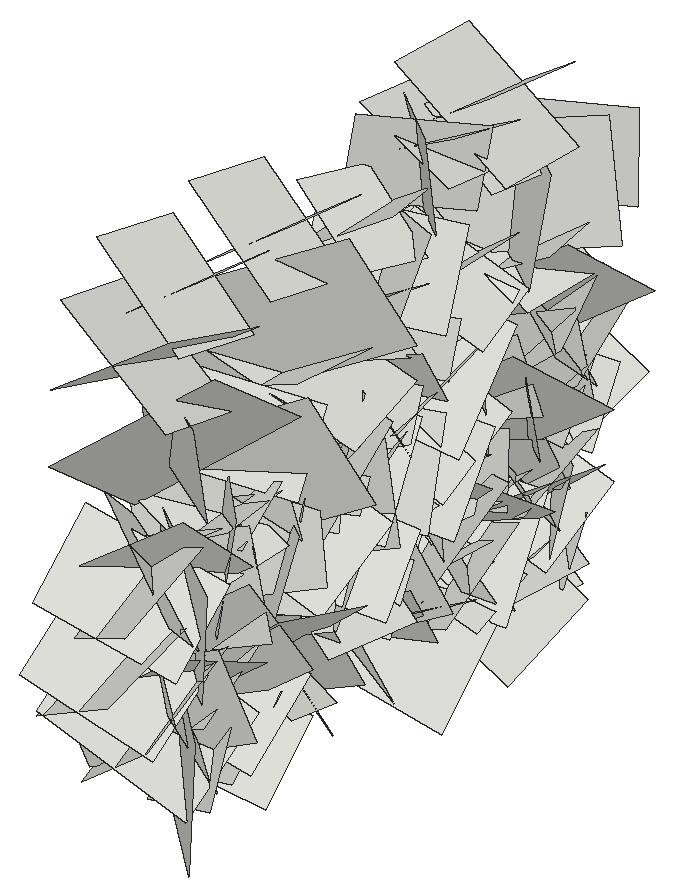
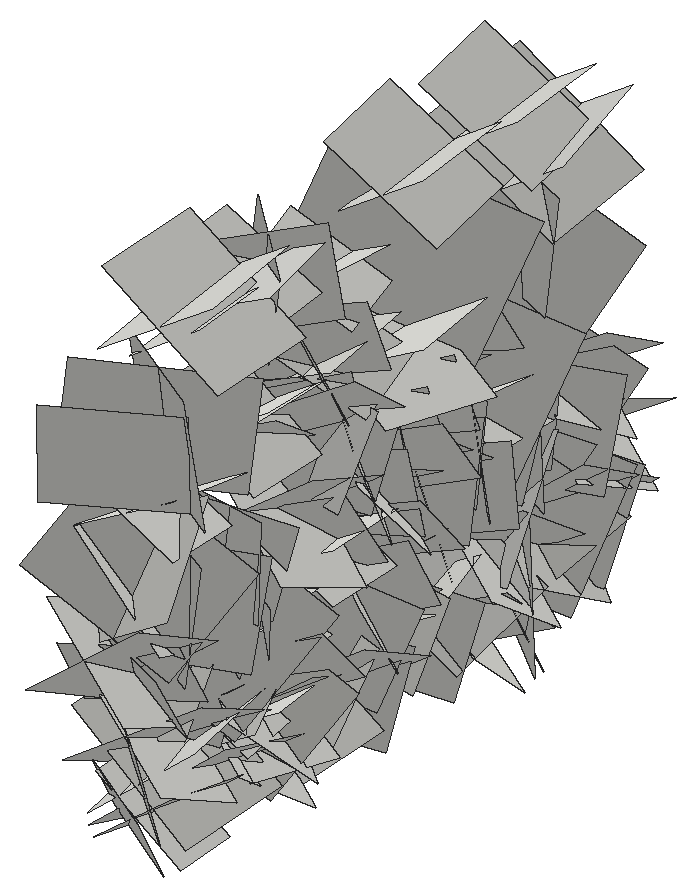
# SketchUp Ruby script. Lengths in inches.
U = 1.inch
M = Sketchup.active_model
def pt(a) = Geom::Point3d.new(a.map { |v| v * U })
def face(e, loops, mat)
  f = e.add_face(loops[0].map { |a| pt(a) })
  loops[1..].each { |l| e.add_face(l.map { |a| pt(a) }).erase! }
  f.material = f.back_material = mat if mat
  f
end
# faces: each face lists its corners as indices into pts; further lists are holes
def faces(e, pts, list, mat = nil) = list.each { |f| face(e, (f[0].is_a?(Array) ? f : [f]).map { |l| l.map { |i| pts[i] } }, mat) }
# xy, xz, yz: faces in a plane at the given z, y or x. An outline is a flat list of corners, or four numbers for a rectangle; further outlines are holes
def ring(l) = l.size == 4 ? [[l[0], l[1]], [l[2], l[1]], [l[2], l[3]], [l[0], l[3]]] : l.each_slice(2).to_a
def flat(e, list, mat, &to3) = list.each { |f| face(e, (f[0].is_a?(Array) ? f : [f]).map { |l| ring(l).map { |u, v| to3.(u, v) } }, mat) }
def xy(e, z, list, mat = nil) = flat(e, list, mat) { |x, y| [x, y, z] }
def xz(e, y, list, mat = nil) = flat(e, list, mat) { |x, z| [x, y, z] }
def yz(e, x, list, mat = nil) = flat(e, list, mat) { |y, z| [x, y, z] }
def lines(e, pts, list) = list.each { |a, b| e.add_line(pt(pts[a]), pt(pts[b])) }
# prism: a flat outline (further loops are holes) pulled along v
def prism(e, loops, v, mat = nil)
  f = face(e, loops, mat); d = Geom::Vector3d.new(v.map { |x| x * U })
  f.pushpull(f.normal.samedirection?(d) ? d.length : -d.length)
end
def box(e, o, s, mat = nil) = prism(e, [[o, [o[0] + s[0], o[1], o[2]], [o[0] + s[0], o[1] + s[1], o[2]], [o[0], o[1] + s[1], o[2]]]], [0, 0, s[2]], mat)
def at(x, y, z, deg = 0) = Geom::Transformation.translation(pt([x, y, z])) * Geom::Transformation.rotation(ORIGIN, Z_AXIS, deg.degrees)
def axes(o, x, y, z) = Geom::Transformation.new([*x, 0, *y, 0, *z, 0, *pt(o).to_a, 1])
def part(name) = M.definitions.add(name)
# library, detail: a bought-in or finely detailed component or shape, given as its bounding box
def library(name, o, s) = part(name).tap { |d| box(d.entities, o, s) }
def detail(e, o, s) = box(e.add_group.entities, o, s)
def put(e, d, t, mat = nil) = e.add_instance(d, t).tap { |i| i.material = mat if mat }
def group(e, t, mat = nil) = e.add_group.tap { |g| g.transformation = t; g.material = mat if mat }.entities
root = M.entities
c1 = part("Component\#6")
p = [[0.01,0,0],[0,3.24,4.54],[4.32,3.24,4.54],[4.33,0,0]]
faces(c1.entities,p,[[0,1,2,3]])
put(root,c1,axes([400.91,128.06,26.23],[-0.10092,-0.80547,-0.37503],[-0.00485,-0.37672,0.81027],[0.94179,-0.08825,-0.03602]))
put(root,c1,axes([404.88,128.06,26.23],[0.10092,-0.80547,-0.37503],[0.00485,-0.37672,0.81027],[-0.94179,-0.08825,-0.03602]))
put(root,c1,axes([400.91,129.13,29.07],[-0.11411,-0.79222,-0.47459],[-0.01099,-0.47673,0.79815],[0.97884,-0.0977,-0.04636]))
put(root,c1,axes([404.88,129.13,29.07],[0.11411,-0.79222,-0.47459],[0.01099,-0.47673,0.79815],[-0.97884,-0.0977,-0.04636]))
put(root,c1,axes([400.91,126.77,21.87],[-0.10992,-0.34124,0.92241],[0.05569,0.92428,0.34784],[1.04103,-0.08548,0.07879]))
put(root,c1,axes([400.91,129.34,35.47],[-0.09463,-0.94647,0.23979],[-0.00571,0.24126,0.95028],[1.03494,-0.08521,0.02717]))
put(root,c1,axes([404.88,129.34,35.47],[0.09463,-0.94647,0.23979],[0.00571,0.24126,0.95028],[-1.03494,-0.08521,0.02717]))
put(root,c1,axes([400.91,130.61,23.63],[-0.04049,-0.92661,-0.53015],[-0.18829,-0.51758,0.91743],[1.11583,-0.12096,0.13557]))
put(root,c1,axes([404.88,130.61,23.63],[0.04049,-0.92661,-0.53015],[0.18829,-0.51758,0.91743],[-1.11583,-0.12096,0.13557]))
put(root,c1,axes([400.91,128.14,26.625],[-0.13018,-0.67547,0.62862],[-0.07474,0.63918,0.67304],[0.97523,-0.04118,0.13549]))
put(root,c1,axes([404.88,128.14,26.625],[0.13018,-0.67547,0.62862],[0.07474,0.63918,0.67304],[-0.97523,-0.04118,0.13549]))
put(root,c1,axes([404.88,126.29,27.49],[0.18614,0.86586,-0.34095],[0.04817,-0.35453,-0.87695],[-0.98523,0.14625,-0.10729]))
put(root,c1,axes([400.91,129.02,36.97],[-0.03047,0.19902,-0.90037],[0.05941,-0.89877,-0.20045],[0.97562,0.06094,-0.01591]))
put(root,c1,axes([400.91,130.54,26.21],[-0.16316,0.13144,-1.2549],[-0.21583,-1.25022,-0.10597],[1.31994,-0.18819,-0.17245]))
put(root,c1,axes([400.91,129.15,30.625],[-0.089,-0.93417,0.70597],[-0.20388,0.70917,0.91554],[1.22433,0.05019,0.20378]))
put(root,c1,axes([400.91,130.09,30.86],[-0.13772,0.10296,-1.023],[-0.01142,-1.03121,-0.10242],[1.08979,0.0022,-0.13035]))
put(root,c1,axes([404.88,130.09,30.86],[0.13772,0.10296,-1.023],[0.01142,-1.03121,-0.10242],[-1.08979,0.0022,-0.13035]))
put(root,c1,axes([400.91,130.39,37.85],[0.05885,-0.83818,0.13983],[-0.03078,0.13818,0.83979],[0.90022,0.05952,0.01957]))
put(root,c1,axes([404.88,130.39,37.85],[-0.05885,-0.83818,0.13983],[0.03078,0.13818,0.83979],[-0.90022,0.05952,0.01957]))
put(root,c1,axes([400.91,128.44,21.53],[-0.07533,-0.68545,1.00594],[-0.30491,0.98857,0.65329],[1.25377,0.19923,0.21932]))
put(root,c1,axes([404.88,128.44,21.53],[0.07533,-0.68545,1.00594],[0.30491,0.98857,0.65329],[-1.25377,0.19923,0.21932]))
put(root,c1,axes([400.91,131.26,22.93],[0.10206,-0.4663,-0.72841],[0.02316,-0.73136,0.47108],[0.91647,0.07041,0.06921]))
put(root,c1,axes([404.88,127.73,24.28],[0.02979,0.75993,0.53946],[0.00151,0.53967,-0.7603],[-0.98786,0.02374,0.0151]))
put(root,c1,axes([400.91,127.73,24.28],[-0.02979,0.75993,0.53946],[-0.00151,0.53967,-0.7603],[0.98786,0.02374,0.0151]))
put(root,c1,axes([400.91,129.03,31.05],[0.04043,0.74356,0.04678],[0.07255,0.04314,-0.74161],[0.78639,-0.04221,0.06601]))
put(root,c1,axes([404.88,129.03,31.05],[-0.04043,0.74356,0.04678],[-0.07255,0.04314,-0.74161],[-0.78639,-0.04221,0.06601]))
put(root,c1,axes([400.91,133.52,31.89],[-0.15087,-0.04242,-1.05475],[-0.23169,-1.04005,0.07132],[1.09469,-0.22597,-0.13027]))
put(root,c1,axes([404.88,133.52,31.89],[0.15087,-0.04242,-1.05475],[0.23169,-1.04005,0.07132],[-1.09469,-0.22597,-0.13027]))
put(root,c1,axes([400.91,129.22,21.54],[-0.01805,0.58513,0.55019],[0.06792,0.54955,-0.58247],[0.84865,-0.03153,0.05832]))
put(root,c1,axes([404.88,129.22,21.54],[0.01805,0.58513,0.55019],[-0.06792,0.54955,-0.58247],[-0.84865,-0.03153,0.05832]))
put(root,c1,axes([404.88,129.75,30.06],[-0.01937,0.49926,0.36665],[-0.0577,0.36409,-0.4985],[-0.65405,-0.04691,0.03312]))
put(root,c1,axes([400.91,130.92,26.67],[-0.06799,-0.20959,0.7931],[0.02884,0.79454,0.21217],[0.86907,-0.04277,0.05501]))
put(root,c1,axes([404.88,130.92,26.67],[0.06799,-0.20959,0.7931],[-0.02884,0.79454,0.21217],[-0.86907,-0.04277,0.05501]))
put(root,c1,axes([400.91,131.21,27.63],[-0.2234,-0.54463,1.08834],[-0.02633,1.10624,0.54877],[1.28976,-0.07175,0.19972]))
put(root,c1,axes([404.88,134.18,33.55],[0.07538,-0.44425,-0.62436],[-0.04133,-0.62833,0.44263],[-0.8112,-0.00926,-0.08057]))
put(root,c1,axes([400.91,134.17,21.91],[-0.00769,-1.04417,0.30366],[-0.13881,0.30229,1.03635],[1.14428,0.02965,0.12776]))
put(root,c1,axes([404.88,134.6875,22.2],[0.10426,-0.66856,0.17597],[-0.06243,0.169,0.67497],[-0.73015,-0.10992,-0.03258]))
put(root,c1,axes([400.91,131.06,25.92],[-0.11704,0.23417,0.88186],[-0.10525,0.87993,-0.24609],[0.96142,0.12483,0.08041]))
put(root,c1,axes([404.88,131.06,25.92],[0.11704,0.23417,0.88186],[0.10525,0.87993,-0.24609],[-0.96142,0.12483,0.08041]))
put(root,c1,axes([400.91,135.18,37.85],[0.05885,-0.83818,0.13983],[-0.03078,0.13818,0.83979],[0.90022,0.05952,0.01957]))
put(root,c1,axes([404.88,135.18,37.85],[-0.05885,-0.83818,0.13983],[0.03078,0.13818,0.83979],[-0.90022,0.05952,0.01957]))
put(root,c1,axes([400.91,133.37,32.625],[-0.2234,-0.54463,1.08834],[-0.02633,1.10624,0.54877],[1.28976,-0.07175,0.19972]))
put(root,c1,axes([400.91,131.97,28.78],[0.10091,0.74431,0.53228],[-0.01265,0.53611,-0.74754],[0.96987,-0.07045,-0.06513]))
put(root,c1,axes([400.91,134.54,24.9375],[0.02484,0.40022,-0.64969],[0.07983,-0.64803,-0.39648],[0.8049,0.05192,0.05937]))
put(root,c1,axes([404.88,134.54,24.9375],[-0.02484,0.40022,-0.64969],[-0.07983,-0.64803,-0.39648],[-0.8049,0.05192,0.05937]))
put(root,c1,axes([404.88,132.79,29.8],[-0.04873,0.29435,0.84438],[0.1159,0.841,-0.28722],[-0.94075,0.08836,-0.07912]))
put(root,c1,axes([400.91,132.79,29.8],[0.04873,0.29435,0.84438],[-0.1159,0.841,-0.28722],[0.94075,0.08836,-0.07912]))
put(root,c1,axes([400.91,133.57,26.39],[-0.0097,-0.16576,1.00827],[-0.11893,1.00238,0.16377],[1.07657,0.10924,0.02717]))
put(root,c1,axes([400.91,132.63,35],[-0.22269,1.01925,0.0867],[0.15354,0.11726,-1.02752],[1.07338,0.19468,0.16497]))
put(root,c1,axes([404.88,132.63,35],[0.22269,1.01925,0.0867],[-0.15354,0.11726,-1.02752],[-1.07338,0.19468,0.16497]))
put(root,c1,axes([400.91,133.77,26.39],[-0.09062,0.64279,0.71838],[0.13606,0.72237,-0.63108],[1.01272,-0.03954,0.14907]))
put(root,c1,axes([400.91,139.12,30.95],[-0.15428,-0.64193,-0.79007],[0.04846,-0.80142,0.64273],[1.07797,-0.05585,-0.14197]))
put(root,c1,axes([404.88,139.12,30.95],[0.15428,-0.64193,-0.79007],[-0.04846,-0.80142,0.64273],[-1.07797,-0.05585,-0.14197]))
put(root,c1,axes([400.91,134.64,27.51],[0.11331,0.92563,-0.03565],[-0.09128,-0.0258,-0.92812],[0.97764,-0.10969,-0.08252]))
put(root,c1,axes([400.91,134.33,29.51],[-0.0444,0.3698,0.86525],[-0.11423,0.85852,-0.37214],[0.99086,0.11554,-0.00413]))
put(root,c1,axes([404.88,134.33,29.51],[0.0444,0.3698,0.86525],[0.11423,0.85852,-0.37214],[-0.99086,0.11554,-0.00413]))
put(root,c1,axes([400.91,139.13,26.61],[-0.02912,-0.4172,-0.72752],[-0.02466,-0.72725,0.41792],[0.88863,-0.03385,-0.01224]))
put(root,c1,axes([404.88,139.13,26.61],[0.02912,-0.4172,-0.72752],[0.02466,-0.72725,0.41792],[-0.88863,-0.03385,-0.01224]))
put(root,c1,axes([400.91,135.78,27.7],[-0.08438,0.31612,0.89331],[0.15155,0.8902,-0.30228],[0.99295,-0.109,0.12205]))
put(root,c1,axes([404.88,138.35,27.1],[0.19626,0.31166,-0.79897],[-0.02742,-0.81497,-0.3239],[-0.90864,0.09191,-0.1628]))
put(root,c1,axes([400.91,137.01,36.4],[0.10049,0.69541,-0.2411],[0.01368,-0.24463,-0.7005],[0.78006,-0.08529,0.04335]))
put(root,c1,axes([404.88,137.01,36.4],[-0.10049,0.69541,-0.2411],[-0.01368,-0.24463,-0.7005],[-0.78006,-0.08529,0.04335]))
put(root,c1,axes([400.91,137.76,20.74],[0.07875,-0.43706,0.66864],[-0.02301,0.67018,0.44047],[0.84643,0.05888,-0.05024]))
put(root,c1,axes([404.88,137.76,20.74],[-0.07875,-0.43706,0.66864],[0.02301,0.67018,0.44047],[-0.84643,0.05888,-0.05024]))
put(root,c1,axes([400.91,139.47,36.72],[0.15825,-0.66033,0.08813],[0.02764,0.09604,0.67542],[0.70562,0.14433,-0.04622]))
put(root,c1,axes([404.88,139.47,36.72],[-0.15825,-0.66033,0.08813],[-0.02764,0.09604,0.67542],[-0.70562,0.14433,-0.04622]))
put(root,c1,axes([400.91,138.53,29.67],[0.03677,-0.4198,0.69058],[0.10131,0.68849,0.41374],[0.85065,-0.06385,-0.07912]))
put(root,c1,axes([404.88,138.53,29.67],[-0.03677,-0.4198,0.69058],[-0.10131,0.68849,0.41374],[-0.85065,-0.06385,-0.07912]))
put(root,c1,axes([404.88,136.92,29.78],[-0.03864,0.57092,0.32429],[0.05823,0.3263,-0.56829],[-0.69355,-0.00442,-0.06578]))
put(root,c1,axes([400.91,137.14,29.31],[0.00249,0.75761,-0.01469],[0.08098,-0.01485,-0.75375],[0.79913,-0.00085,0.07643]))
put(root,c1,axes([404.88,137.14,29.31],[-0.00249,0.75761,-0.01469],[-0.08098,-0.01485,-0.75375],[-0.79913,-0.00085,0.07643]))
put(root,c1,axes([400.91,135.48,23.28],[-0.21581,1.04519,0.5846],[-0.09636,0.57779,-1.06467],[1.26577,0.22219,0.01862]))
put(root,c1,axes([404.88,141.16,33.73],[-0.01034,-0.20439,-0.70125],[0.11317,-0.69418,0.20085],[-0.76594,-0.09981,0.03914]))
put(root,c1,axes([404.88,137.77,24.11],[0.1419,0.78136,-0.16109],[-0.04598,-0.15597,-0.79258],[-0.84441,0.13979,0.01609]))
put(root,c1,axes([400.91,137.53,34.5],[-0.08019,0.3809,0.76753],[0.04804,0.77121,-0.37826],[0.90698,-0.00717,0.08789]))
put(root,c1,axes([404.88,137.53,34.5],[0.08019,0.3809,0.76753],[-0.04804,0.77121,-0.37826],[-0.90698,-0.00717,0.08789]))
put(root,c1,axes([400.91,136.3,32.46],[-0.17238,0.91042,0.71253],[-0.07022,0.71102,-0.92361],[1.22345,0.16908,0.04738]))
put(root,c1,axes([400.91,137.68,27.62],[0.00267,0.49736,0.77514],[0.05686,0.77375,-0.49665],[0.97459,-0.04651,0.02685]))
put(root,c1,axes([404.88,137.85,30.84],[0.06669,0.91948,0.38333],[0.06841,0.37952,-0.92095],[-1.05374,0.08283,-0.03553]))
put(root,c1,axes([400.91,137.85,30.84],[-0.06669,0.91948,0.38333],[-0.06841,0.37952,-0.92095],[1.05374,0.08283,-0.03553]))
put(root,c1,axes([404.88,143.53,22.21],[0.15224,-0.84766,-0.36991],[0.10957,-0.35729,0.85887],[-0.97421,-0.17265,0.03879]))
put(root,c1,axes([400.91,139.84,37.375],[0.13047,0.02824,0.77],[-0.11824,0.77221,-0.01049],[0.80815,0.10842,-0.12584]))
put(root,c1,axes([404.88,139.84,37.375],[-0.13047,0.02824,0.77],[0.11824,0.77221,-0.01049],[-0.80815,0.10842,-0.12584]))
put(root,c1,axes([400.91,143.38,25.93],[-0.00088,-0.66729,0.07011],[0.1194,0.06898,0.65784],[0.70113,-0.01259,-0.11194]))
put(root,c1,axes([404.88,143.38,25.93],[0.00088,-0.66729,0.07011],[-0.1194,0.06898,0.65784],[-0.70113,-0.01259,-0.11194]))
put(root,c1,axes([404.88,144.18,33.46],[0.08879,-0.56105,-0.39599],[-0.0694,-0.40364,0.55803],[-0.72461,-0.03009,-0.10197]))
put(root,c1,axes([400.91,144.6,22.65],[-0.17478,-0.82558,-0.09028],[0.09417,-0.10904,0.83495],[0.87528,-0.15312,-0.10786]))
put(root,c1,axes([404.88,144.6,22.65],[0.17478,-0.82558,-0.09028],[-0.09417,-0.10904,0.83495],[-0.87528,-0.15312,-0.10786]))
put(root,c1,axes([400.91,145.12,23.07],[-0.0526,-0.82286,-0.58821],[0.0059,-0.58914,0.82367],[1.07215,-0.03713,-0.03339]))
put(root,c1,axes([400.91,145.6875,25.3],[-0.21495,-0.77208,-0.77151],[-0.06755,-0.77499,0.79232],[1.15499,-0.18901,-0.09724]))
put(root,c1,axes([404.88,145.6875,25.3],[0.21495,-0.77208,-0.77151],[0.06755,-0.77499,0.79232],[-1.15499,-0.18901,-0.09724]))
put(root,c1,axes([400.91,140.84,40.56],[-0.05261,0.712,-0.12967],[0.10362,-0.12219,-0.70833],[0.7601,0.06594,0.08758]))
put(root,c1,axes([404.88,140.84,40.56],[0.05261,0.712,-0.12967],[-0.10362,-0.12219,-0.70833],[-0.7601,0.06594,0.08758]))
put(root,c1,axes([404.88,144.73,33.27],[0.16555,-0.76551,-0.15352],[-0.02389,-0.16091,0.77946],[-0.82725,-0.14855,-0.05323]))
put(root,c1,axes([400.91,140.76,35.5625],[0.0095,0.80566,-0.00603],[-0.04784,-0.00552,-0.80445],[0.85268,-0.00929,-0.04507]))
put(root,c1,axes([404.88,140.76,35.5625],[-0.0095,0.80566,-0.00603],[0.04784,-0.00552,-0.80445],[-0.85268,-0.00929,-0.04507]))
put(root,c1,axes([400.91,143.64,28.51],[0.01569,-0.00258,-0.72773],[0.02057,-0.72762,0.00297],[0.77112,0.01947,0.01473]))
put(root,c1,axes([404.88,143.64,28.51],[-0.01569,-0.00258,-0.72773],[-0.02057,-0.72762,0.00297],[-0.77112,0.01947,0.01473]))
put(root,c1,axes([400.91,141.61,27.46],[-0.15544,0.8369,-0.58263],[-0.03072,-0.5918,-0.84279],[1.08048,0.10358,-0.10778]))
put(root,c1,axes([404.88,141.61,27.46],[0.15544,0.8369,-0.58263],[0.03072,-0.5918,-0.84279],[-1.08048,0.10358,-0.10778]))
put(root,c1,axes([400.91,144.76,23.61],[0.10873,-0.7568,0.02149],[-0.01122,0.02025,0.76368],[0.80245,0.10283,0.00777]))
put(root,c1,axes([404.88,144.76,23.61],[-0.10873,-0.7568,0.02149],[0.01122,0.02025,0.76368],[-0.80245,0.10283,0.00777]))
put(root,c1,axes([400.91,144.05,31.85],[-0.11078,0.17753,-0.74918],[0.12323,-0.74375,-0.19246],[0.80677,0.13798,-0.07348]))
put(root,c1,axes([404.88,144.05,31.85],[0.11078,0.17753,-0.74918],[-0.12323,-0.74375,-0.19246],[-0.80677,0.13798,-0.07348]))
put(root,c1,axes([400.91,145.42,24.52],[-0.2647,-0.88765,0.75819],[-0.01358,0.77738,0.90589],[1.23735,-0.18136,0.17214]))
put(root,c1,axes([400.91,141.63,23.18],[-0.01995,1.00092,0.30572],[-0.13829,0.30114,-0.99396],[1.10071,0.05598,-0.11933]))
put(root,c1,axes([404.88,145.72,37.21],[-0.0202,-0.65006,0.07365],[0.02062,0.07308,0.65011],[-0.69316,0.02112,0.01719]))
put(root,c1,axes([404.88,142.67,41.25],[0.05619,0.9574,-0.08237],[-0.00834,-0.08206,-0.95886],[-1.01856,0.05349,0.00331]))
put(root,c1,axes([400.91,142.67,41.25],[-0.05619,0.9574,-0.08237],[0.00834,-0.08206,-0.95886],[1.01856,0.05349,0.00331]))
put(root,c1,axes([404.88,145.6,27.28],[-0.00806,0.29423,-0.56577],[-0.12293,-0.55701,-0.28812],[-0.6647,0.09945,0.06014]))
put(root,c1,axes([400.91,147.86,21.63],[-0.08807,-1.00346,0.13322],[-0.11481,0.14172,0.99989],[1.06685,-0.06759,0.1186]))
put(root,c1,axes([404.88,147.86,21.63],[0.08807,-1.00346,0.13322],[0.11481,0.14172,0.99989],[-1.06685,-0.06759,0.1186]))
put(root,c1,axes([404.88,146.3,23.53],[0.0913,-0.50535,0.50896],[-0.05568,0.5068,0.51209],[-0.75823,-0.09807,0.02368]))
put(root,c1,axes([400.91,147.08,31.53],[-0.0186,0.21399,-0.90436],[-0.04027,-0.90393,-0.21315],[0.98427,-0.03294,-0.02581]))
put(root,c1,axes([404.88,147.08,31.53],[0.0186,0.21399,-0.90436],[0.04027,-0.90393,-0.21315],[-0.98427,-0.03294,-0.02581]))
put(root,c1,axes([400.91,144.98,23.12],[0.11015,0.70988,0.06167],[-0.04855,0.06885,-0.71532],[0.75374,-0.09931,-0.05509]))
put(root,c1,axes([404.88,144.98,23.12],[-0.11015,0.70988,0.06167],[0.04855,0.06885,-0.71532],[-0.75374,-0.09931,-0.05509]))
put(root,c1,axes([404.88,149.13,24.11],[0.03147,-0.85153,-0.39996],[0.02133,-0.3995,0.85202],[-0.997,-0.03542,0.00561]))
put(root,c1,axes([400.91,149.13,24.11],[-0.03147,-0.85153,-0.39996],[-0.02133,-0.3995,0.85202],[0.997,-0.03542,0.00561]))
put(root,c1,axes([400.91,144.71,33.13],[-0.16995,0.04512,1.05289],[-0.00982,1.0649,-0.04705],[1.11704,0.01623,0.15977]))
put(root,c1,axes([404.88,144.71,33.13],[0.16995,0.04512,1.05289],[0.00982,1.0649,-0.04705],[-1.11704,0.01623,0.15977]))
put(root,c1,axes([400.91,148.52,32.35],[0.08011,-0.79067,-0.06214],[0.07476,-0.05548,0.79163],[0.83736,0.0806,-0.06473]))
put(root,c1,axes([404.88,148.52,32.35],[-0.08011,-0.79067,-0.06214],[-0.07476,-0.05548,0.79163],[-0.83736,0.0806,-0.06473]))
put(root,c1,axes([400.91,149.17,29.19],[0.22051,-0.77582,-0.34275],[-0.07369,-0.36732,0.78924],[0.89602,0.16072,0.14925]))
put(root,c1,axes([400.91,146.7,34.04],[-0.22474,0.77203,-0.6543],[-0.03576,-0.67353,-0.78378],[1.07212,0.13937,-0.1633]))
put(root,c1,axes([404.88,146.7,34.04],[0.22474,0.77203,-0.6543],[0.03576,-0.67353,-0.78378],[-1.07212,0.13937,-0.1633]))
put(root,c1,axes([404.88,145.7,22.51],[0.08358,0.19729,0.79599],[0.0899,0.79341,-0.20506],[-0.86462,0.10156,0.05562]))
put(root,c1,axes([404.88,146.45,21.25],[0.00375,0.2874,0.54008],[-0.0654,0.5375,-0.28562],[-0.64519,-0.05282,0.03209]))
put(root,c1,axes([400.91,149.44,28.46],[-0.01637,-0.35652,-0.61871],[0.18604,-0.60176,0.34238],[0.7337,0.14463,-0.10062]))
put(root,c1,axes([404.88,149.44,28.46],[0.01637,-0.35652,-0.61871],[-0.18604,-0.60176,0.34238],[-0.7337,0.14463,-0.10062]))
put(root,c1,axes([400.91,150.98,27.43],[0.11329,-0.77541,-0.3635],[-0.07754,-0.37325,0.77469],[0.90445,0.06513,0.11195]))
put(root,c1,axes([404.88,150.98,27.43],[-0.11329,-0.77541,-0.3635],[0.07754,-0.37325,0.77469],[-0.90445,0.06513,0.11195]))
put(root,c1,axes([404.88,150.44,37.52],[0.01758,-0.03984,-0.83316],[-0.08726,-0.82933,0.03802],[-0.87984,0.08145,-0.02042]))
